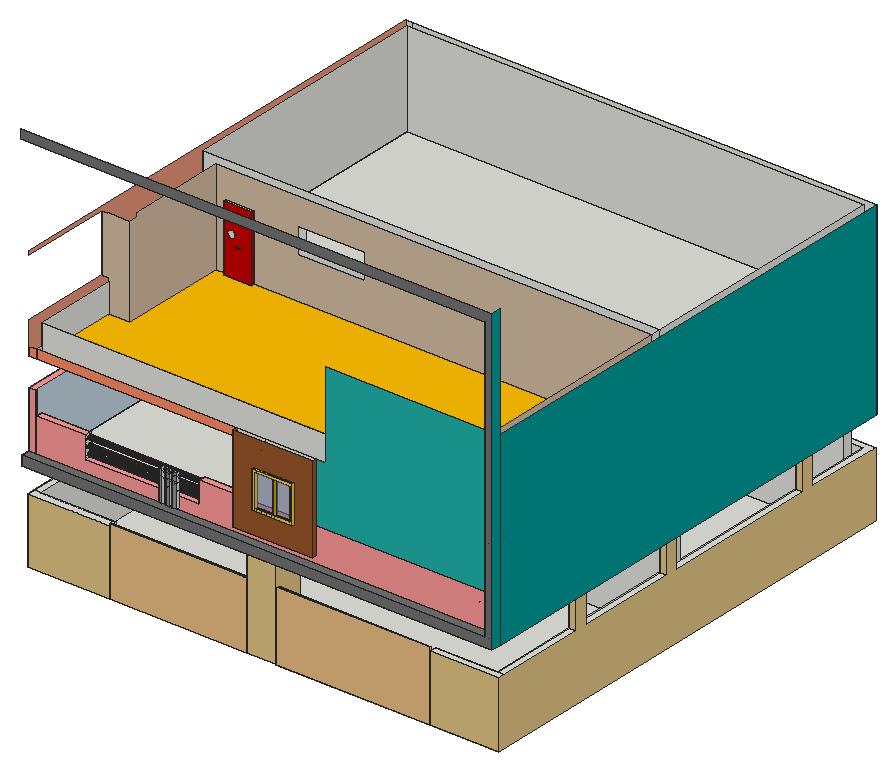
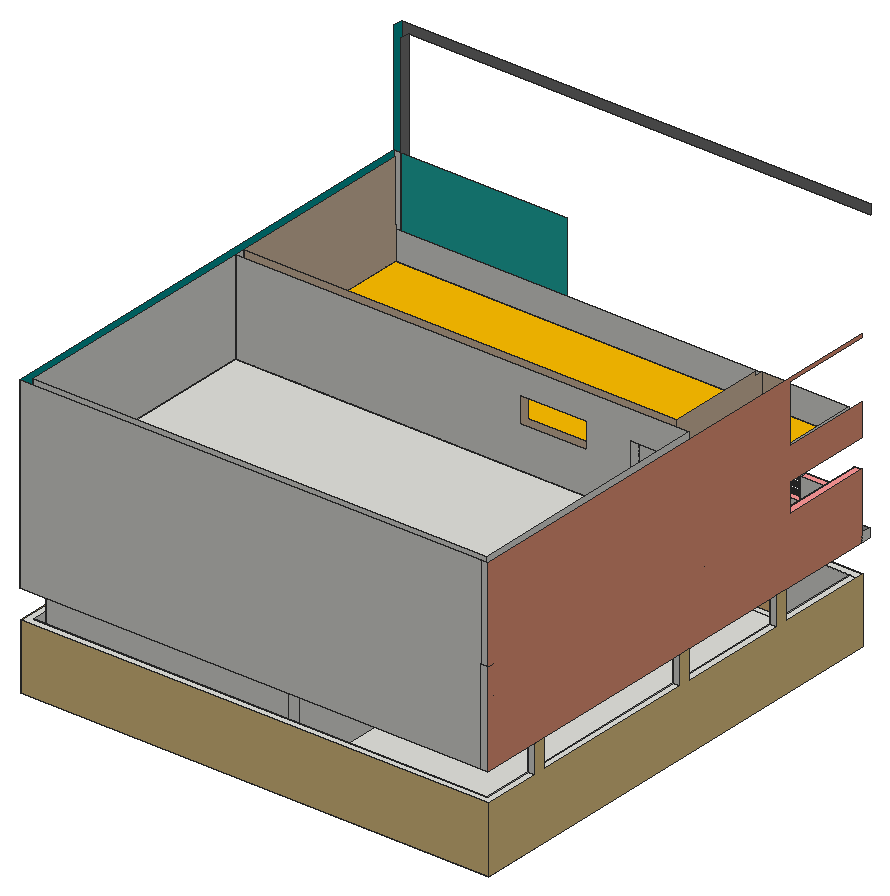
# SketchUp Ruby script. Lengths in inches.
U = 1.inch
M = Sketchup.active_model
def pt(a) = Geom::Point3d.new(a.map { |v| v * U })
def face(e, loops, mat)
  f = e.add_face(loops[0].map { |a| pt(a) })
  loops[1..].each { |l| e.add_face(l.map { |a| pt(a) }).erase! }
  f.material = f.back_material = mat if mat
  f
end
# faces: each face lists its corners as indices into pts; further lists are holes
def faces(e, pts, list, mat = nil) = list.each { |f| face(e, (f[0].is_a?(Array) ? f : [f]).map { |l| l.map { |i| pts[i] } }, mat) }
# xy, xz, yz: faces in a plane at the given z, y or x. An outline is a flat list of corners, or four numbers for a rectangle; further outlines are holes
def ring(l) = l.size == 4 ? [[l[0], l[1]], [l[2], l[1]], [l[2], l[3]], [l[0], l[3]]] : l.each_slice(2).to_a
def flat(e, list, mat, &to3) = list.each { |f| face(e, (f[0].is_a?(Array) ? f : [f]).map { |l| ring(l).map { |u, v| to3.(u, v) } }, mat) }
def xy(e, z, list, mat = nil) = flat(e, list, mat) { |x, y| [x, y, z] }
def xz(e, y, list, mat = nil) = flat(e, list, mat) { |x, z| [x, y, z] }
def yz(e, x, list, mat = nil) = flat(e, list, mat) { |y, z| [x, y, z] }
def lines(e, pts, list) = list.each { |a, b| e.add_line(pt(pts[a]), pt(pts[b])) }
# prism: a flat outline (further loops are holes) pulled along v
def prism(e, loops, v, mat = nil)
  f = face(e, loops, mat); d = Geom::Vector3d.new(v.map { |x| x * U })
  f.pushpull(f.normal.samedirection?(d) ? d.length : -d.length)
end
def box(e, o, s, mat = nil) = prism(e, [[o, [o[0] + s[0], o[1], o[2]], [o[0] + s[0], o[1] + s[1], o[2]], [o[0], o[1] + s[1], o[2]]]], [0, 0, s[2]], mat)
def at(x, y, z, deg = 0) = Geom::Transformation.translation(pt([x, y, z])) * Geom::Transformation.rotation(ORIGIN, Z_AXIS, deg.degrees)
def axes(o, x, y, z) = Geom::Transformation.new([*x, 0, *y, 0, *z, 0, *pt(o).to_a, 1])
def part(name) = M.definitions.add(name)
# library, detail: a bought-in or finely detailed component or shape, given as its bounding box
def library(name, o, s) = part(name).tap { |d| box(d.entities, o, s) }
def detail(e, o, s) = box(e.add_group.entities, o, s)
def put(e, d, t, mat = nil) = e.add_instance(d, t).tap { |i| i.material = mat if mat }
def group(e, t, mat = nil) = e.add_group.tap { |g| g.transformation = t; g.material = mat if mat }.entities
root = M.entities
M.materials.add("[0014_DarkSalmon]").color = [233, 150, 122]
M.materials.add("[0082_LightSeaGreen]").color = [32, 178, 170]
M.materials.add("[Color A02]").color = [255, 153, 153]
M.materials.add("[Color A06]").color = [204, 0, 0]
M.materials.add("[Color B02]").color = [255, 178, 153]
M.materials.add("[Color B03]").color = [255, 140, 101]
M.materials.add("[Color B07]").color = [153, 38, 0]
M.materials.add("[Color D04]").color = [255, 204, 50]
M.materials.add("[Color D05]").color = [255, 191, 0]
M.materials.add("[Color D06]").color = [204, 153, 0]
M.materials.add("[Color H07]").color = [0, 153, 153]
M.materials.add("[Color M04]").color = [142, 142, 142]
M.materials.add("[Color M05]").color = [114, 114, 114]
M.materials.add("[Formica Laminate Light]").color = [213, 189, 164]
M.materials.add("[Stone Brushed Khaki]").color = [226, 197, 133]
M.materials.add("[Terrazzo Light Blue]").color = [196, 214, 227]
M.materials.add("[Translucent Glass Sky Reflection]").color = [126, 138, 183]
M.materials["[Translucent Glass Sky Reflection]"].alpha = 0.52
M.materials.add("[Translucent Glass Tinted]").color = [8, 201, 241]
M.materials["[Translucent Glass Tinted]"].alpha = 0.48
M.materials.add("[Wood Cherry Original]").color = [152, 86, 42]
c1 = library("Modern+Gate+1",[0,0,0],[118.11,1.97,78.74])
xy(root,0,[[1.35,10.95,1.35,610.95,601.35,610.95,601.35,10.95,513.07,10.95,513.07,19.95,592.35,19.95,592.35,301.18,592.5625,301.18,592.5625,309.99,592.35,309.99,592.35,601.95,10.35,601.95,10.35,19.95,105.28,19.95,105.28,10.95],[105.28,10.95,280.34,19.95],[280.34,10.95,317.41,48.18],[317.41,10.95,513.07,19.95],[10.35,19.95,280.34,19.95,280.34,48.18,317.41,48.18,317.41,19.95,592.35,19.95,592.35,301.18,280.34,301.18,280.34,582.81,592.03,582.81,592.03,572.24,294.72,572.24,294.72,310.12,317.41,310.12,317.41,309.99,592.35,309.99,592.35,601.95,10.35,601.95],
  [280.34,301.18,280.34,319.74,294.53,319.74,294.53,310.12,294.72,310.12,294.72,309.87,317.41,309.87,317.41,301.18],[317.41,301.18,592.35,301.56],[592.35,301.18,592.5625,301.56],[317.41,301.56,592.35,309.99],[592.35,301.56,592.5625,309.99],
  [294.72,309.87,317.41,310.12],[294.53,310.12,294.72,319.74],[280.34,319.74,294.72,564.24],[280.34,564.24,280.34,582.81,317.41,582.81,317.41,572.24,294.72,572.24,294.72,564.24],[317.41,572.24,592.03,582.81]])
xy(root,84,[[1.35,10.95,105.28,19.95],[513.07,10.95,601.35,19.95],[1.35,19.95,10.35,134.07],[592.35,19.95,601.35,134.07],[1.35,148.63,10.35,289.57],
  [592.35,148.63,601.35,148.63,601.35,278.74,592.5625,278.74,592.5625,293.31,601.35,293.31,601.35,495.33,592.64,495.33,592.64,509.9,601.35,509.9,601.35,610.95,1.35,610.95,1.35,536.26,10.35,536.26,10.35,601.95,592.35,601.95],[1.35,304.13,10.35,521.7]])
xy(root,120,[[280.34,10.95,317.41,48.18],[1.35,134.07,10.35,148.63],[592.35,134.07,601.35,148.63],[592.5625,278.74,601.35,293.31],[601.35,278.74,601.5625,293.31],
  [1.35,289.57,10.35,304.13],[280.34,301.18,592.5625,301.18,592.5625,309.99,317.41,309.99,317.41,309.87,294.72,309.87,294.72,310.12,294.53,310.12,294.53,319.74,294.72,319.74,294.72,572.24,592.03,572.24,592.03,582.81,280.34,582.81],[294.72,309.87,317.41,310.12],[294.53,310.12,294.72,319.74],[592.64,495.33,601.35,509.9],
  [601.35,495.33,601.64,509.9],[1.35,521.7,10.35,536.26]])
xy(root,120.8,[[1.5625,0,1.5625,612,11.0625,612,11.0625,603,10.5625,603,10.5625,11.9375,592.5625,11.9375,592.5625,12,596.75,12,596.75,0],[596.75,0,601.625,12],[10.5625,11.9375,11.0625,12],[11.0625,11.9375,35.5625,12],[35.5625,11.9375,592.5625,12],
  [10.5625,12,11.0625,21],[11.0625,12,592.5625,21],[592.5625,12,592.5625,603,11.0625,603,11.0625,612,601.5625,612,601.5625,12],[10.5625,21,11.0625,277.84],[11.0625,21,592.5625,21,592.5625,277.84,85.5,277.84,85.5,274.84,49.5,274.84,49.5,277.84,11.0625,277.84],
  [49.5,274.84,85.5,277.84],[10.5625,277.84,11.0625,603],[11.0625,277.84,592.5625,603]])
xy(root,132.61,[[1.5625,0,592.5625,12]],"[Color M05]")
xy(root,133.86,[[168.95,8.9375,173.39,11.9375],[178.14,8.9375,182.89,11.9375],[186.14,8.9375,191.95,11.9375]])
xy(root,141.3,[[265.96,12,301.8125,13.5],[301.8125,12,367.5,13.5]])
xy(root,141.3,[[265.96,6,367.6875,12]],"[Wood Cherry Original]")
xy(root,147.61,[[73.56,11.9375,218.56,21]],"[Color A02]")
xy(root,153.17,[[57.91,271.84,70.66,274.84]])
xy(root,155.11,[[57.91,271.84,70.66,274.84]],"[Color A02]")
xy(root,162.11,[[265.96,12,592.5625,12,592.5625,21,269.07,21]])
xy(root,170.84,[[293.09,3,343.9,6]],"[Color D04]")
xy(root,173.84,[[318.49,5,322.39,6]])
xy(root,173.84,[[296.09,3,318.49,6],[318.49,3,322.39,5],[322.39,3,340.9,6]],"[Color D04]")
xy(root,174.68,[[181.96,274.84,184.61,277.84]],"[Color B07]")
xy(root,175.18,[[168.95,8.9375,173.39,11.9375]])
xy(root,175.36,[[10.5625,11.9375,73.56,21],[218.56,11.9375,592.5625,11.9375,592.5625,12,265.96,12,269.07,21,218.56,21]],"[Color A02]")
xy(root,175.59,[[186.14,8.9375,191.95,11.9375]])
xy(root,175.67,[[178.14,8.9375,182.89,11.9375]])
xy(root,204.8,[[10.5625,12,11.0625,127.99],[49.5,274.84,85.5,277.84]])
xy(root,204.8,[[1.5625,12,10.5625,127.99]],"[Color A02]")
xy(root,207.74,[[181.96,274.84,184.61,277.84]],"[Color B07]")
xy(root,215.4,[[318.49,5,322.39,6]])
xy(root,215.4,[[296.09,3,318.49,6],[318.49,3,322.39,5],[322.39,3,340.9,6]],"[Color D04]")
xy(root,218.4,[[293.09,3,343.9,6]],"[Color D04]")
xy(root,240.8,[[1.5625,12,1.5625,127.99,10.5625,127.99,10.5625,20.9375,11.0625,20.9375,11.0625,12],[10.5625,20.9375,11.0625,21],[11.0625,20.9375,592.5625,21],[10.5625,21,10.6875,127.99],[11.0625,21,592.5625,21.5],
  [10.5625,127.99,36.75,265.15],[49.5,262.15,85.5,265.15],[10.5625,265.15,36.75,277.84],[36.75,265.15,49.5,277.84],[49.5,265.15,85.5,277.84],
  [85.5,265.15,592.5625,277.84],[10.5625,277.84,592.5625,603]])
xy(root,240.8,[[11.0625,21.5,592.5625,21.5,592.5625,265.15,85.5,265.15,85.5,262.15,49.5,262.15,49.5,265.15,36.75,265.15,36.75,127.99,11.0625,127.99]],"[Color D05]")
xz(root,0,[[1.5625,120.8,601.625,120.8,601.625,504.72,0,504.72,0,492.8,592.5625,492.8,592.5625,132.61,1.5625,132.61]],"[Color M05]")
xz(root,3,[[[293.09,170.84,343.9,218.4],[296.09,173.84,340.9,215.4]]],"[Color D04]")
xz(root,5,[[318.49,173.84,322.39,215.4]],"[Color D06]")
xz(root,6,[[[293.09,170.84,343.9,218.4],[296.09,173.84,340.9,215.4]],[318.49,173.84,322.39,215.4]])
xz(root,6,[[296.09,173.84,318.49,215.4],[322.39,173.84,340.9,215.4]],"[Translucent Glass Sky Reflection]")
xz(root,6,[[[265.96,141.3,367.6875,251.61],[293.09,170.84,343.9,218.4]]],"[Wood Cherry Original]")
xz(root,8.9375,[[168.95,133.86,173.39,175.18],[178.14,133.86,182.89,175.67],[186.14,133.86,191.95,175.59]],"[Color M04]")
xz(root,10.95,[[1.35,0,105.28,84],[280.34,0,317.41,120],[513.07,0,601.35,84]],"[Stone Brushed Khaki]")
xz(root,11.9375,[[168.95,133.86,173.39,147.61],[178.14,133.86,182.89,147.61],[186.14,133.86,191.95,147.61],[168.95,147.61,173.39,175.18],[178.14,147.61,182.89,175.67],
  [186.14,147.61,191.95,175.59]])
xz(root,11.9375,[[10.5625,120.8,592.5625,120.8,592.5625,175.36,218.56,175.36,218.56,147.61,191.95,147.61,191.95,133.86,186.14,133.86,186.14,147.61,182.89,147.61,182.89,133.86,178.14,133.86,178.14,147.61,173.39,147.61,173.39,133.86,168.95,133.86,168.95,147.61,73.56,147.61,73.56,175.36,10.5625,175.36]],"[Color A02]")
xz(root,12,[[10.5625,120.8,35.5625,132.61],[35.5625,120.8,592.5625,132.61],[592.5625,120.8,596.75,132.61],[596.75,120.8,601.5625,240.8],[601.5625,120.8,601.625,240.8],
  [592.5625,132.61,596.75,132.61,596.75,240.8,601.5625,240.8,601.5625,360.8,592.5625,360.8],[265.96,141.3,301.8125,162.11],[301.8125,141.3,367.5,162.11],[367.5,141.3,367.6875,162.11],[10.5625,162.11,11.0625,204.8],
  [265.96,162.11,301.8125,175.36],[301.8125,162.11,367.5,175.36],[367.5,162.11,367.6875,175.36],[367.6875,162.11,592.5625,175.36],[265.96,175.36,367.5,240.8],
  [367.5,175.36,367.6875,240.8],[265.96,240.8,301.8125,251.61],[301.8125,240.8,367.6875,251.61],[601.5625,240.8,601.625,504.72]])
xz(root,12,[[367.6875,175.36,592.5625,175.36,592.5625,360.8,380.39,360.8,380.39,251.61,367.6875,251.61]],"[0082_LightSeaGreen]")
xz(root,12,[[1.5625,132.61,10.5625,204.8]],"[Color A02]")
xz(root,12,[[1.5625,240.8,11.0625,251.61],[11.0625,240.8,265.96,251.61]],"[Color B03]")
xz(root,13.5,[[265.96,129.33,367.5,141.3]])
xz(root,19.95,[[10.35,0,105.28,84],[513.07,0,592.35,84]])
xz(root,20.9375,[[10.5625,240.8,592.5625,277.61]])
xz(root,21,[[10.5625,120.8,10.5625,175.36,73.56,175.36,73.56,147.61,218.56,147.61,218.56,175.36,269.07,175.36,269.07,162.11,592.5625,162.11,592.5625,120.8],[10.5625,240.8,10.6875,277.61],[10.6875,240.8,592.5625,277.61]])
xz(root,48.18,[[280.34,0,317.41,120]])
xz(root,127.99,[[10.5625,204.8,11.0625,240.8],[10.5625,240.8,10.6875,277.61]])
xz(root,127.99,[[1.5625,204.8,10.5625,240.8]],"[Color A02]")
xz(root,127.99,[[10.6875,240.8,36.75,240.8,36.75,355.8,10.5625,355.8,10.5625,355.61,1.5625,355.61,1.5625,282.11,10.5625,282.11,10.5625,277.61,10.6875,277.61]],"[Formica Laminate Light]")
xz(root,134.07,[[1.35,84,10.35,120]])
xz(root,134.07,[[592.35,84,601.35,120]],"[Stone Brushed Khaki]")
xz(root,148.63,[[1.35,84,10.35,120]])
xz(root,148.63,[[592.35,84,601.35,120]],"[Stone Brushed Khaki]")
xz(root,262.15,[[[49.5,240.8,85.5,324.8],[59.23,285.14,57.91,285.3125,56.67,285.82,55.61,286.64,54.79,287.7,54.28,288.9375,54.11,290.26,54.28,291.59,54.79,292.82,55.61,293.89,56.67,294.7,57.91,295.21,59.23,295.39,60.56,295.21,61.8,294.7,62.86,293.89,63.67,292.82,64.18,291.59,64.36,290.26,64.18,288.9375,63.67,287.7,62.86,286.64,61.8,285.82,60.56,285.3125],[61.8125,275.45,72.25,278.01]]],"[Color A06]")
xz(root,265.15,[[10.5625,240.8,36.75,324.8],[49.5,240.8,85.5,324.8]])
xz(root,265.15,[[[36.75,240.8,49.5,240.8,49.5,324.8,85.5,324.8,85.5,240.8,592.5625,240.8,592.5625,360.8,36.75,360.8],[141.83,294.68,227.4,327.74]]],"[Formica Laminate Light]")
xz(root,271.84,[[57.91,153.17,70.66,155.11]],"[Color A02]")
xz(root,271.84,[[57.91,162.47,59.57,162.6875,61.125,163.33,62.46,164.35,63.48,165.6875,64.125,167.24,64.34,168.91,64.125,170.57,63.48,172.125,62.46,173.46,61.125,174.48,59.57,175.125,57.91,175.34,56.24,175.125,54.6875,174.48,53.35,173.46,52.33,172.125,51.6875,170.57,51.47,168.91,51.6875,167.24,52.33,165.6875,53.35,164.35,54.6875,163.33,56.24,162.6875]],"[Color B02]")
xz(root,274.84,[[57.91,153.17,70.66,155.11],[57.91,162.47,56.24,162.6875,54.6875,163.33,53.35,164.35,52.33,165.6875,51.6875,167.24,51.47,168.91,51.6875,170.57,52.33,172.125,53.35,173.46,54.6875,174.48,56.24,175.125,57.91,175.34,59.57,175.125,61.125,174.48,62.46,173.46,63.48,172.125,64.125,170.57,64.34,168.91,64.125,167.24,63.48,165.6875,62.46,164.35,61.125,163.33,59.57,162.6875]])
xz(root,274.84,[[[49.5,120.8,85.5,204.8],[57.91,162.47,56.24,162.6875,54.6875,163.33,53.35,164.35,52.33,165.6875,51.6875,167.24,51.47,168.91,51.6875,170.57,52.33,172.125,53.35,173.46,54.6875,174.48,56.24,175.125,57.91,175.34,59.57,175.125,61.125,174.48,62.46,173.46,63.48,172.125,64.125,170.57,64.34,168.91,64.125,167.24,63.48,165.6875,62.46,164.35,61.125,163.33,59.57,162.6875],[57.91,153.17,70.66,155.11]]],"[Color A06]")
xz(root,274.84,[[181.96,174.68,184.61,207.74]],"[Color B07]")
xz(root,277.84,[[49.5,120.8,85.5,204.8],[181.96,174.68,184.61,207.74],[[10.5625,240.8,10.5625,360.8,592.5625,360.8,592.5625,240.8,85.5,240.8,85.5,324.8,49.5,324.8,49.5,240.8],[141.83,294.68,227.4,327.74]]])
xz(root,277.84,[[[10.5625,120.8,49.5,120.8,49.5,204.8,85.5,204.8,85.5,120.8,592.5625,120.8,592.5625,240.8,10.5625,240.8],[141.83,174.68,227.4,207.74]]],"[Terrazzo Light Blue]")
xz(root,277.84,[[141.83,174.68,161.89,191.21],[161.89,174.68,181.96,191.21],[184.61,174.68,206,191.21],[206,174.68,227.4,191.21],[141.83,191.21,161.89,207.74],
  [161.89,191.21,181.96,207.74],[184.61,191.21,206,207.74],[206,191.21,227.4,207.74]],"[Translucent Glass Tinted]")
xz(root,278.74,[[592.5625,84,601.35,120]],"[Stone Brushed Khaki]")
xz(root,289.57,[[1.35,84,10.35,120]])
xz(root,293.31,[[592.5625,84,601.35,120]],"[Stone Brushed Khaki]")
xz(root,301.18,[[280.34,0,592.5625,120]])
xz(root,304.13,[[1.35,84,10.35,120]])
xz(root,309.87,[[294.72,0,317.41,120]])
xz(root,309.99,[[317.41,0,592.5625,120]])
xz(root,310.12,[[294.53,0,294.72,120],[294.72,0,317.41,120]])
xz(root,495.33,[[592.64,84,601.35,120]],"[Stone Brushed Khaki]")
xz(root,509.9,[[592.64,84,601.35,120]],"[Stone Brushed Khaki]")
xz(root,521.7,[[1.35,84,10.35,120]])
xz(root,536.26,[[1.35,84,10.35,120]])
xz(root,572.24,[[294.72,0,592.03,120]])
xz(root,582.81,[[280.34,0,592.03,120]])
xz(root,601.95,[[10.35,0,592.35,84]])
xz(root,603,[[10.5625,120.8,592.5625,240.8],[10.5625,240.8,592.5625,360.8]])
xz(root,610.95,[[1.35,0,601.35,84]],"[Stone Brushed Khaki]")
xz(root,612,[[1.5625,120.8,11.0625,240.8],[11.0625,120.8,601.5625,360.8],[1.5625,240.8,11.0625,360.8]])
yz(root,1.35,[[10.95,0,10.95,84,134.07,84,134.07,120,148.63,120,148.63,84,289.57,84,289.57,120,304.13,120,304.13,84,521.7,84,521.7,120,536.26,120,536.26,84,610.95,84,610.95,0]],"[Stone Brushed Khaki]")
yz(root,1.5625,[[0,120.8,12,132.61]])
yz(root,1.5625,[[12,120.8,12,204.8,127.99,204.8,127.99,240.8,12,240.8,12,282.11,127.99,282.11,127.99,355.8,12,355.8,12,360.8,612,360.8,612,120.8]],"[0014_DarkSalmon]")
yz(root,10.35,[[19.95,0,601.95,0,601.95,84,536.26,84,536.26,120,521.7,120,521.7,84,304.13,84,304.13,120,289.57,120,289.57,84,148.63,84,148.63,120,134.07,120,134.07,84,19.95,84]])
yz(root,10.5625,[[11.9375,120.8,11.9375,175.36,12,132.61,12,120.8],[12,120.8,21,175.36],[277.84,120.8,603,240.8],[12,132.61,11.9375,175.36,12,175.36],[20.9375,240.8,21,277.61],
  [21,240.8,127.99,277.61],[265.15,240.8,277.84,324.8],[277.84,240.8,603,360.8]])
yz(root,10.5625,[[21,120.8,277.84,120.8,277.84,240.8,127.99,240.8,127.99,204.8,12,204.8,12,175.36,21,175.36]],"[Terrazzo Light Blue]")
yz(root,10.6875,[[21,240.8,127.99,277.61]])
yz(root,11.0625,[[12,240.8,21.5,251.61]])
yz(root,36.75,[[127.99,240.8,265.15,240.8,265.15,360.8,139.1875,360.8,139.1875,355.8,127.99,355.8]],"[Formica Laminate Light]")
yz(root,49.5,[[274.84,120.8,277.84,204.8],[262.15,240.8,265.15,324.8],[265.15,240.8,277.84,324.8]])
yz(root,57.91,[[271.84,153.17,274.84,155.11]])
yz(root,70.66,[[271.84,153.17,274.84,155.11]])
yz(root,73.56,[[11.9375,147.61,11.97,147.61,11.97,151.86,11.9375,175.36],[[11.98,147.61,21,147.61,21,175.36,11.9375,175.36,11.97,151.86],[16.84,168.93,16.16,169.02,15.52,169.28,14.98,169.7,14.5625,170.24,14.3,170.875,14.21,171.55,14.3,172.23,14.5625,172.87,14.98,173.41,15.52,173.83,16.16,174.09,16.84,174.18,17.52,174.09,18.15,173.83,18.69,173.41,19.11,172.87,19.37,172.23,19.46,171.55,19.37,170.875,19.11,170.24,18.69,169.7,18.15,169.28,17.52,169.02],[16.84,158.99,16.16,159.08,15.52,159.34,14.98,159.76,14.5625,160.3,14.3,160.9375,14.21,161.62,14.3,162.3,14.5625,162.93,14.98,163.47,15.52,163.89,16.16,164.15,16.84,164.24,17.52,164.15,18.15,163.89,18.69,163.47,19.11,162.93,19.37,162.3,19.46,161.62,19.37,160.9375,19.11,160.3,18.69,159.76,18.15,159.34,17.52,159.08],[16.84,150.37,16.16,150.46,15.52,150.72,14.98,151.14,14.5625,151.68,14.3,152.3125,14.21,152.99,14.3,153.67,14.5625,154.3,14.98,154.85,15.52,155.27,16.16,155.53,16.84,155.62,17.52,155.53,18.15,155.27,18.69,154.85,19.11,154.3,19.37,153.67,19.46,152.99,19.37,152.3125,19.11,151.68,18.69,151.14,18.15,150.72,17.52,150.46]],[11.97,147.61,11.98,147.61,11.97,151.86],[16.84,150.37,16.16,150.46,15.52,150.72,14.98,151.14,14.5625,151.68,14.3,152.3125,14.21,152.99,14.3,153.67,14.5625,154.3,14.98,154.85,15.52,155.27,16.16,155.53,16.84,155.62,17.52,155.53,18.15,155.27,18.69,154.85,19.11,154.3,19.37,153.67,19.46,152.99,19.37,152.3125,19.11,151.68,18.69,151.14,18.15,150.72,17.52,150.46]])
yz(root,85.5,[[274.84,120.8,277.84,204.8],[265.15,240.8,277.84,324.8]])
yz(root,85.5,[[262.15,240.8,265.15,324.8]],"[Color A06]")
yz(root,105.28,[[10.95,0,19.95,84]])
yz(root,168.95,[[8.9375,133.86,11.9375,175.18]])
yz(root,173.39,[[8.9375,133.86,11.9375,175.18]])
yz(root,178.14,[[8.9375,133.86,11.9375,175.67]])
yz(root,181.96,[[274.84,174.68,277.84,207.74]],"[Color B07]")
yz(root,182.89,[[8.9375,133.86,11.9375,175.67]])
yz(root,184.61,[[274.84,174.68,277.84,207.74]],"[Color B07]")
yz(root,186.14,[[8.9375,133.86,11.9375,175.59]])
yz(root,191.95,[[8.9375,133.86,11.9375,175.59]])
yz(root,218.06,[[16.84,150.37,17.52,150.46,18.15,150.72,18.69,151.14,19.11,151.68,19.37,152.3125,19.46,152.99,19.37,153.67,19.11,154.3,18.69,154.85,18.15,155.27,17.52,155.53,16.84,155.62,16.16,155.53,15.52,155.27,14.98,154.85,14.5625,154.3,14.3,153.67,14.21,152.99,14.3,152.3125,14.5625,151.68,14.98,151.14,15.52,150.72,16.16,150.46]])
yz(root,218.56,[[11.9375,147.61,21,175.36]])
yz(root,221.31,[[16.84,168.93,17.52,169.02,18.15,169.28,18.69,169.7,19.11,170.24,19.37,170.875,19.46,171.55,19.37,172.23,19.11,172.87,18.69,173.41,18.15,173.83,17.52,174.09,16.84,174.18,16.16,174.09,15.52,173.83,14.98,173.41,14.5625,172.87,14.3,172.23,14.21,171.55,14.3,170.875,14.5625,170.24,14.98,169.7,15.52,169.28,16.16,169.02]])
yz(root,223.68,[[16.84,158.99,17.52,159.08,18.15,159.34,18.69,159.76,19.11,160.3,19.37,160.9375,19.46,161.62,19.37,162.3,19.11,162.93,18.69,163.47,18.15,163.89,17.52,164.15,16.84,164.24,16.16,164.15,15.52,163.89,14.98,163.47,14.5625,162.93,14.3,162.3,14.21,161.62,14.3,160.9375,14.5625,160.3,14.98,159.76,15.52,159.34,16.16,159.08]])
yz(root,265.96,[[6,141.3,12,251.61]],"[Wood Cherry Original]")
yz(root,280.34,[[301.18,0,319.74,120],[319.74,0,564.24,120],[564.24,0,582.81,120]])
yz(root,280.34,[[10.95,0,48.18,120]],"[Stone Brushed Khaki]")
yz(root,293.09,[[3,170.84,6,218.4]],"[Color D04]")
yz(root,294.72,[[309.87,0,310.12,120],[310.12,0,572.24,120]])
yz(root,296.09,[[3,173.84,6,215.4]],"[Color D04]")
yz(root,317.41,[[309.87,0,309.99,120],[309.99,0,310.12,120]])
yz(root,317.41,[[10.95,0,48.18,120]],"[Stone Brushed Khaki]")
yz(root,318.49,[[5,173.84,6,215.4]],"[Color D06]")
yz(root,322.39,[[5,173.84,6,215.4]],"[Color D06]")
yz(root,340.9,[[3,173.84,6,215.4]],"[Color D04]")
yz(root,343.9,[[3,170.84,6,218.4]],"[Color D04]")
yz(root,367.6875,[[6,141.3,12,251.61]],"[Wood Cherry Original]")
yz(root,513.07,[[10.95,0,19.95,84]])
yz(root,592.03,[[572.24,0,582.81,120]])
yz(root,592.35,[[19.95,0,19.95,84,134.07,84,134.07,120,148.63,120,148.63,84,601.95,84,601.95,0]])
yz(root,592.5625,[[301.18,0,301.56,120],[301.56,0,309.99,120],[278.74,84,293.31,120],[11.9375,120.8,12,132.61],[12,120.8,21,162.11],
  [277.84,120.8,603,240.8],[11.9375,132.61,12,175.36],[12,162.11,21,240.8],[20.9375,240.8,21,277.61],[265.15,240.8,277.84,360.8],
  [277.84,240.8,603,360.8]])
yz(root,592.5625,[[0,132.61,0,492.8,12,492.8,12,175.36,11.9375,175.36,11.9375,132.61]],"[Color M05]")
yz(root,592.5625,[[21,240.8,21,282.11,21.5,282.11,21.5,360.8,265.15,360.8,265.15,240.8]],"[Formica Laminate Light]")
yz(root,592.5625,[[21,120.8,277.84,240.8]],"[Terrazzo Light Blue]")
yz(root,592.64,[[495.33,84,509.9,120]])
yz(root,601.35,[[10.95,0,610.95,0,610.95,84,509.9,84,509.9,120,495.33,120,495.33,84,293.31,84,293.31,120,278.74,120,278.74,84,148.63,84,148.63,120,134.07,120,134.07,84,10.95,84]],"[Stone Brushed Khaki]")
yz(root,601.5625,[[12,120.8,612,360.8]],"[Color H07]")
yz(root,601.625,[[0,120.8,12,504.72]],"[Color H07]")
p = [[73.56,16.84,150.37],[218.06,16.84,150.37],[218.06,16.16,150.46],[73.56,16.16,150.46],[73.56,17.52,150.46],[218.06,17.52,150.46],
  [218.06,15.52,150.72],[73.56,15.52,150.72],[73.56,18.15,150.72],[218.06,18.15,150.72],[218.06,14.98,151.14],[73.56,14.98,151.14],
  [73.56,18.69,151.14],[218.06,18.69,151.14],[218.06,14.5625,151.68],[73.56,14.5625,151.68],[73.56,19.11,151.68],[218.06,19.11,151.68],
  [218.06,14.3,152.3125],[73.56,14.3,152.3125],[73.56,19.37,152.3125],[218.06,19.37,152.3125],[218.06,14.21,152.99],[73.56,14.21,152.99],
  [73.56,19.46,152.99],[218.06,19.46,152.99],[218.06,14.3,153.67],[73.56,14.3,153.67],[73.56,19.37,153.67],[218.06,19.37,153.67],
  [218.06,14.5625,154.3],[73.56,14.5625,154.3],[73.56,19.11,154.3],[218.06,19.11,154.3],[218.06,14.98,154.85],[73.56,14.98,154.85],
  [73.56,18.69,154.85],[218.06,18.69,154.85],[218.06,15.52,155.27],[73.56,15.52,155.27],[73.56,18.15,155.27],[218.06,18.15,155.27],
  [218.06,16.16,155.53],[73.56,16.16,155.53],[73.56,17.52,155.53],[218.06,17.52,155.53],[218.06,16.84,155.62],[73.56,16.84,155.62],
  [73.56,16.16,159.08],[73.56,16.84,158.99],[223.68,16.84,158.99],[223.68,16.16,159.08],[73.56,17.52,159.08],[223.68,17.52,159.08],
  [73.56,15.52,159.34],[223.68,15.52,159.34],[73.56,18.15,159.34],[223.68,18.15,159.34],[73.56,14.98,159.76],[223.68,14.98,159.76],
  [73.56,18.69,159.76],[223.68,18.69,159.76],[73.56,14.5625,160.3],[223.68,14.5625,160.3],[73.56,19.11,160.3],[223.68,19.11,160.3],
  [73.56,14.3,160.9375],[223.68,14.3,160.9375],[73.56,19.37,160.9375],[223.68,19.37,160.9375],[73.56,14.21,161.62],[223.68,14.21,161.62],
  [73.56,19.46,161.62],[223.68,19.46,161.62],[73.56,14.3,162.3],[223.68,14.3,162.3],[73.56,19.37,162.3],[223.68,19.37,162.3],
  [265.96,12,162.11],[269.07,21,162.11],[269.07,21,175.36],[265.96,12,175.36],[73.56,14.5625,162.93],[223.68,14.5625,162.93],
  [73.56,19.11,162.93],[223.68,19.11,162.93],[56.24,274.84,162.6875],[57.91,274.84,162.47],[57.91,271.84,162.47],[56.24,271.84,162.6875],
  [59.57,274.84,162.6875],[59.57,271.84,162.6875],[54.6875,274.84,163.33],[54.6875,271.84,163.33],[61.125,274.84,163.33],[61.125,271.84,163.33],
  [73.56,14.98,163.47],[223.68,14.98,163.47],[73.56,18.69,163.47],[223.68,18.69,163.47],[53.35,274.84,164.35],[53.35,271.84,164.35],
  [62.46,274.84,164.35],[62.46,271.84,164.35],[73.56,15.52,163.89],[223.68,15.52,163.89],[73.56,18.15,163.89],[223.68,18.15,163.89],
  [73.56,16.16,164.15],[223.68,16.16,164.15],[73.56,17.52,164.15],[223.68,17.52,164.15],[73.56,16.84,164.24],[223.68,16.84,164.24],
  [52.33,274.84,165.6875],[52.33,271.84,165.6875],[63.48,274.84,165.6875],[63.48,271.84,165.6875],[51.6875,274.84,167.24],[51.6875,271.84,167.24],
  [64.125,274.84,167.24],[64.125,271.84,167.24],[51.47,274.84,168.91],[51.47,271.84,168.91],[64.34,274.84,168.91],[64.34,271.84,168.91],
  [73.56,16.16,169.02],[73.56,16.84,168.93],[221.31,16.84,168.93],[221.31,16.16,169.02],[73.56,17.52,169.02],[221.31,17.52,169.02],
  [51.6875,274.84,170.57],[51.6875,271.84,170.57],[64.125,274.84,170.57],[64.125,271.84,170.57],[73.56,15.52,169.28],[221.31,15.52,169.28],
  [73.56,18.15,169.28],[221.31,18.15,169.28],[73.56,14.98,169.7],[221.31,14.98,169.7],[73.56,18.69,169.7],[221.31,18.69,169.7],
  [73.56,14.5625,170.24],[221.31,14.5625,170.24],[73.56,19.11,170.24],[221.31,19.11,170.24],[73.56,14.3,170.875],[221.31,14.3,170.875],
  [73.56,19.37,170.875],[221.31,19.37,170.875],[52.33,274.84,172.125],[52.33,271.84,172.125],[63.48,274.84,172.125],[63.48,271.84,172.125],
  [73.56,14.21,171.55],[221.31,14.21,171.55],[73.56,19.46,171.55],[221.31,19.46,171.55],[73.56,14.3,172.23],[221.31,14.3,172.23],
  [73.56,19.37,172.23],[221.31,19.37,172.23],[53.35,274.84,173.46],[53.35,271.84,173.46],[62.46,274.84,173.46],[62.46,271.84,173.46],
  [73.56,14.5625,172.87],[221.31,14.5625,172.87],[73.56,19.11,172.87],[221.31,19.11,172.87],[73.56,14.98,173.41],[221.31,14.98,173.41],
  [73.56,18.69,173.41],[221.31,18.69,173.41],[73.56,15.52,173.83],[221.31,15.52,173.83],[73.56,18.15,173.83],[221.31,18.15,173.83],
  [54.6875,274.84,174.48],[54.6875,271.84,174.48],[61.125,274.84,174.48],[61.125,271.84,174.48],[73.56,16.16,174.09],[221.31,16.16,174.09],
  [73.56,17.52,174.09],[221.31,17.52,174.09],[73.56,16.84,174.18],[221.31,16.84,174.18],[56.24,274.84,175.125],[56.24,271.84,175.125],
  [59.57,274.84,175.125],[59.57,271.84,175.125],[57.91,274.84,175.34],[57.91,271.84,175.34],[10.5625,603,204.8],[1.5625,603,204.8],
  [10.5625,603,240.8],[1.5625,603,240.8],[10.5625,265.15,204.8],[1.5625,265.15,204.8],[1.5625,612,240.8],[601.5625,21.5,240.8],
  [592.5625,21.5,240.8],[301.8125,12,240.8],[301.8125,6,240.8],[367.5,12,129.33],[367.6875,12,129.33],[367.5,13.5,129.33],
  [265.96,12,129.33],[265.96,13.5,129.33],[596.75,12,240.8],[596.75,0,240.8],[596.75,12,132.61],[596.75,0,132.61]]
faces(root,p,[[0,1,2,3],[4,5,1,0],[3,2,6,7],[8,9,5,4],[7,6,10,11],[12,13,9,8],[11,10,14,15],[16,17,13,12],
  [15,14,18,19],[20,21,17,16],[19,18,22,23],[24,25,21,20],[23,22,26,27],[28,29,25,24],[27,26,30,31],[32,33,29,28],
  [31,30,34,35],[36,37,33,32],[35,34,38,39],[40,41,37,36],[39,38,42,43],[44,45,41,40],[43,42,46,47],[47,46,45,44],
  [48,49,50,51],[49,52,53,50],[54,48,51,55],[52,56,57,53],[58,54,55,59],[56,60,61,57],[62,58,59,63],[60,64,65,61],
  [66,62,63,67],[64,68,69,65],[70,66,67,71],[68,72,73,69],[74,70,71,75],[72,76,77,73],[82,74,75,83],[76,84,85,77],
  [96,82,83,97],[84,98,99,85],[104,96,97,105],[98,106,107,99],[108,104,105,109],[106,110,111,107],[112,108,109,113],[110,112,113,111],
  [126,127,128,129],[127,130,131,128],[136,126,129,137],[130,138,139,131],[140,136,137,141],[138,142,143,139],[144,140,141,145],[142,146,147,143],
  [148,144,145,149],[146,150,151,147],[156,148,149,157],[150,158,159,151],[160,156,157,161],[158,162,163,159],[168,160,161,169],[162,170,171,163],
  [172,168,169,173],[170,174,175,171],[176,172,173,177],[174,178,179,175],[184,176,177,185],[178,186,187,179],[188,184,185,189],[186,188,189,187]],"[Color A06]")
faces(root,p,[[78,79,80,81]])
faces(root,p,[[86,87,88,89],[87,90,91,88],[92,86,89,93],[90,94,95,91],[100,92,93,101],[94,102,103,95],[114,100,101,115],[102,116,117,103],
  [118,114,115,119],[116,120,121,117],[122,118,119,123],[120,124,125,121],[132,122,123,133],[124,134,135,125],[152,132,133,153],[134,154,155,135],
  [164,152,153,165],[154,166,167,155],[180,164,165,181],[166,182,183,167],[190,180,181,191],[182,192,193,183],[194,190,191,195],[192,194,195,193]],"[Color B02]")
lines(root,p,[[196,197],[198,199],[200,201],[199,202],[203,204],[205,206],[207,208],[207,209],[210,211],[212,213],[214,215]])
put(root,c1,axes([105.28,10.77,0],[1.48327,0,0],[0,1.09,0],[0,0,1.09]))
put(root,c1,axes([317.41,10.71,0],[1.65614,0,0],[0,1.12,0],[0,0,1.12]))
